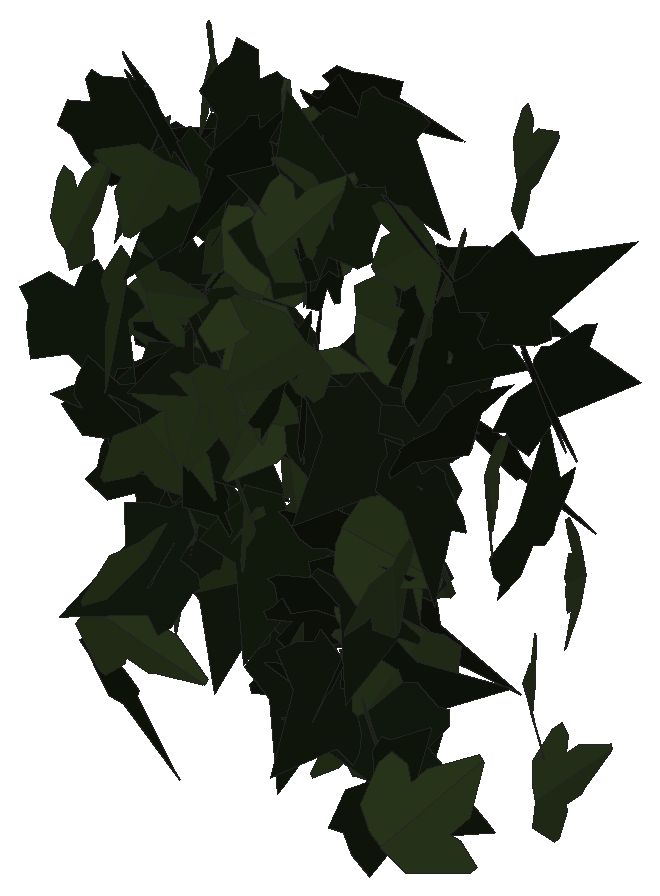
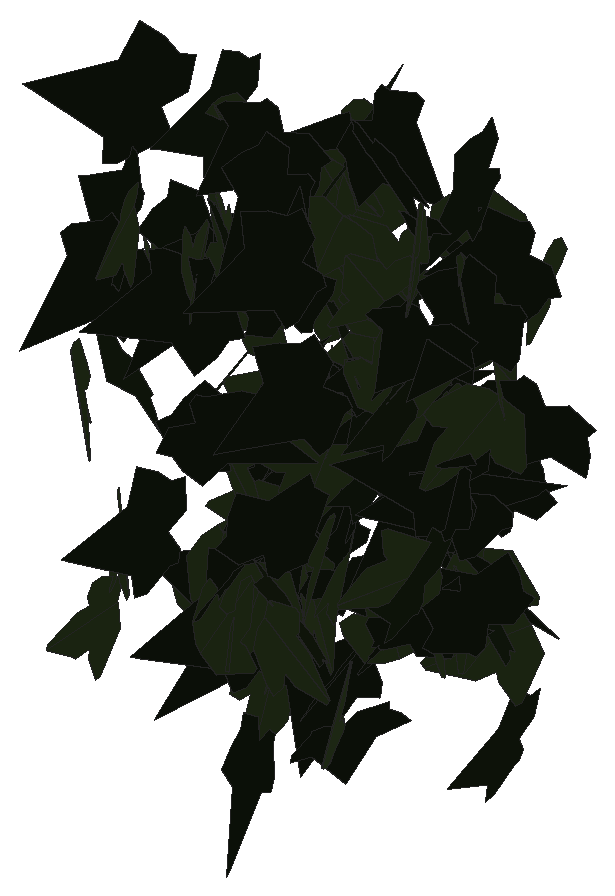
# SketchUp Ruby script. Lengths in inches.
U = 1.inch
M = Sketchup.active_model
def pt(a) = Geom::Point3d.new(a.map { |v| v * U })
def face(e, loops, mat)
  f = e.add_face(loops[0].map { |a| pt(a) })
  loops[1..].each { |l| e.add_face(l.map { |a| pt(a) }).erase! }
  f.material = f.back_material = mat if mat
  f
end
# faces: each face lists its corners as indices into pts; further lists are holes
def faces(e, pts, list, mat = nil) = list.each { |f| face(e, (f[0].is_a?(Array) ? f : [f]).map { |l| l.map { |i| pts[i] } }, mat) }
# xy, xz, yz: faces in a plane at the given z, y or x. An outline is a flat list of corners, or four numbers for a rectangle; further outlines are holes
def ring(l) = l.size == 4 ? [[l[0], l[1]], [l[2], l[1]], [l[2], l[3]], [l[0], l[3]]] : l.each_slice(2).to_a
def flat(e, list, mat, &to3) = list.each { |f| face(e, (f[0].is_a?(Array) ? f : [f]).map { |l| ring(l).map { |u, v| to3.(u, v) } }, mat) }
def xy(e, z, list, mat = nil) = flat(e, list, mat) { |x, y| [x, y, z] }
def xz(e, y, list, mat = nil) = flat(e, list, mat) { |x, z| [x, y, z] }
def yz(e, x, list, mat = nil) = flat(e, list, mat) { |y, z| [x, y, z] }
def lines(e, pts, list) = list.each { |a, b| e.add_line(pt(pts[a]), pt(pts[b])) }
# prism: a flat outline (further loops are holes) pulled along v
def prism(e, loops, v, mat = nil)
  f = face(e, loops, mat); d = Geom::Vector3d.new(v.map { |x| x * U })
  f.pushpull(f.normal.samedirection?(d) ? d.length : -d.length)
end
def box(e, o, s, mat = nil) = prism(e, [[o, [o[0] + s[0], o[1], o[2]], [o[0] + s[0], o[1] + s[1], o[2]], [o[0], o[1] + s[1], o[2]]]], [0, 0, s[2]], mat)
def at(x, y, z, deg = 0) = Geom::Transformation.translation(pt([x, y, z])) * Geom::Transformation.rotation(ORIGIN, Z_AXIS, deg.degrees)
def axes(o, x, y, z) = Geom::Transformation.new([*x, 0, *y, 0, *z, 0, *pt(o).to_a, 1])
def part(name) = M.definitions.add(name)
# library, detail: a bought-in or finely detailed component or shape, given as its bounding box
def library(name, o, s) = part(name).tap { |d| box(d.entities, o, s) }
def detail(e, o, s) = box(e.add_group.entities, o, s)
def put(e, d, t, mat = nil) = e.add_instance(d, t).tap { |i| i.material = mat if mat }
def group(e, t, mat = nil) = e.add_group.tap { |g| g.transformation = t; g.material = mat if mat }.entities
root = M.entities
M.materials.add("efeu1").color = [18, 25, 13]
M.materials.add("efeu2").color = [43, 57, 29]
c1 = part("ivyleaf_9")
p = [[1.54,2.16,1.25],[1.36,2.04,1.19],[-0.21,0.99,0.68],[-0.71,1.11,0.82],[-0.85,0.86,0.67],[-0.8,0.17,0.21],
  [-0.9,-0.01,0.1],[-0.67,-0.16,-0.02],[-0.08,-0.08,-0.05],[-0.03,-0.6,-0.4],[0.65,-0.88,-0.66],[0.83,-0.6,-0.49],
  [1.29,-0.42,-0.43],[1.8125,-0.07,-0.26],[1.21,0.44,0.15]]
faces(c1.entities,p,[[0,1,2,3,4,5,6,7,8,9,10,11,12,13,14]],"efeu1")
c2 = part("ivyleaf_10")
p = [[0,0.5,-0.03],[-0.0625,2.02,-0.43],[-0.19,2.01,-0.46],[-0.54,1.05,-0.29],[-0.52,0.625,-0.18],[-0.83,0.76,-0.28],
  [-1.16,0.64,-0.33],[-1.15,0.33,-0.24],[-0.77,-0.39,0.02],[-0.3,-0.51,0.16],[0.04,-0.48,0.23],[-0.02,2.01,-0.4375],
  [-0.06,2.01,-0.43],[0.04,-0.49,0.23],[0.67,-0.49,0.14],[1.38,0.36,-0.2],[1.375,0.51,-0.24],[0.81,0.65,-0.19],
  [0.62,0.59,-0.15],[0.6,1.09,-0.28],[0.5,1.23,-0.31]]
faces(c2.entities,p,[[0,1,2,3,4,5,6,7,8,9,10],[11,12,0,13,14,15,16,17,18,19,20]],"efeu2")
put(root,c1,axes([535.21,138.35,177.43],[0.48207,-0.59856,0.20369],[0.14027,-0.14851,-0.76839],[0.61651,0.50182,0.01555]))
put(root,c1,axes([535.3125,134.73,179.44],[-0.27899,-0.26925,-0.74167],[0.55413,0.49316,-0.38748],[0.56171,-0.62025,0.01388]))
put(root,c1,axes([535.34,135.23,182.82],[0.09988,-0.00032,-0.76274],[0.56999,0.51119,0.07443],[0.50683,-0.57483,0.06661]))
put(root,c1,axes([535.74,135.73,181.85],[0.51801,0.54955,0.22927],[0.14515,0.17819,-0.75505],[-0.5775,0.53773,0.01588]))
put(root,c2,axes([536.02,133.7,181.36],[0.0294,0.29057,-0.75135],[0.02416,0.75119,0.29146],[0.80521,-0.03315,0.01869]))
put(root,c1,axes([535.76,135.85,175.4],[-0.15333,-0.07864,0.76423],[0.70864,0.28655,0.17166],[-0.29677,0.72488,0.01505]))
put(root,c2,axes([535.86,137.66,177.16],[0.10862,0.11928,0.73924],[0.24864,0.69886,-0.1493],[-0.70632,0.26435,0.06113]))
put(root,c2,axes([536.05,135.42,181.02],[0.22066,-0.82498,0.09562],[-0.00156,0.09853,0.85365],[-0.83051,-0.21937,0.0238]))
put(root,c1,axes([535.81,134.89,172.53],[0.60317,-0.5162,0.04875],[0.03688,-0.03188,-0.7939],[0.51719,0.6043,-0.00024]))
put(root,c2,axes([536.13,135.38,179.3],[-0.52269,-0.40509,-0.52109],[0.39164,0.34468,-0.6608],[0.53127,-0.65264,-0.02555]))
put(root,c1,axes([536.88,135.8,177.53],[-0.42085,-0.08815,0.66579],[-0.62736,-0.22886,-0.42686],[0.23972,-0.75367,0.05175]))
put(root,c2,axes([536.5,135.43,182],[0.32264,-0.70335,-0.12966],[-0.06803,0.11142,-0.77367],[0.71196,0.32939,-0.01517]))
put(root,c1,axes([536.52,135.94,178.05],[0.62655,0.0255,-0.47755],[-0.4781,0.01515,-0.62647],[-0.01109,0.78765,0.02751]))
put(root,c1,axes([536.25,136.89,181.72],[-0.24445,-0.32961,-0.64417],[0.44367,0.46886,-0.40827],[0.57163,-0.50486,0.04141]))
put(root,c2,axes([536.68,136.55,183.5],[0.32496,-0.53129,-0.4965],[-0.05851,0.52295,-0.59789],[0.72482,0.28041,0.17433]))
put(root,c2,axes([536.27,134.6875,179.95],[0.26676,-0.48349,0.71737],[0.51173,-0.51709,-0.5388],[0.69751,0.56427,0.12093]))
put(root,c1,axes([536.1875,134.58,177.1],[-0.17328,0.05557,0.77942],[0.69673,-0.35045,0.17988],[0.35376,0.71743,0.0275]))
put(root,c1,axes([536.24,135.2,177.59],[0.4585,0.2321,0.66706],[0.55433,0.37457,-0.51134],[-0.43767,0.71756,0.05116]))
put(root,c1,axes([536.91,134.43,174.72],[-0.55418,0.52698,-0.25199],[-0.19513,0.16039,0.76454],[0.55058,0.58728,0.01732]))
put(root,c1,axes([537.2,136.13,174.625],[-0.6712,-0.43181,0.12924],[0.11128,0.0659,0.79809],[-0.43678,0.68034,0.00472]))
put(root,c1,axes([536.28,135.96,178.14],[0.41914,-0.00437,0.67662],[0.66741,0.13362,-0.41257],[-0.11133,0.78462,0.07403]))
put(root,c1,axes([536.67,134.73,183.85],[0.79047,-0.33972,-0.29967],[-0.27706,0.11427,-0.86037],[0.3584,0.83761,-0.00417]))
put(root,c1,axes([536.55,137.02,180.19],[0.60846,-0.46082,0.01006],[0.00814,-0.00592,-0.76327],[0.46086,0.60851,0.0002]))
put(root,c2,axes([537.34,134.36,182.62],[-0.64774,-0.28277,0.33722],[-0.29999,-0.15534,-0.70649],[0.322,-0.71356,0.02017]))
put(root,c2,axes([537.07,134.3125,175.25],[-0.32956,-0.7796,-0.26398],[0.09485,0.24649,-0.84636],[0.8176,-0.34284,-0.00822]))
put(root,c2,axes([536.7,134.04,174.02],[-0.50139,-0.05608,-0.73277],[0.72865,0.07765,-0.50451],[0.09576,-0.88448,0.00217]))
put(root,c1,axes([537.71,134.34,175.34],[-0.77582,0.09988,0.22816],[-0.22554,0.03492,-0.7822],[-0.10566,-0.80792,-0.0056]))
put(root,c2,axes([537.16,138.5,173.49],[-0.43688,0.49632,0.37938],[0.23325,-0.29987,0.6609],[0.57953,0.49484,0.01999]))
put(root,c2,axes([536.98,135.62,174.79],[0.14997,-0.35752,0.68886],[0.48487,-0.50468,-0.36749],[0.60602,0.49227,0.12355]))
put(root,c1,axes([537.0625,135.8,180.34],[0.16986,-0.77294,0.08753],[0.03334,-0.08228,-0.79125],[0.77717,0.17246,0.01481]))
put(root,c1,axes([537.21,135.625,177.28],[0.07653,-0.30387,-0.73011],[-0.08193,0.72653,-0.31096],[0.78657,0.10524,0.03864]))
put(root,c2,axes([537.34,134.36,177.6],[-0.58863,-0.52168,-0.42239],[0.3064,0.29103,-0.78643],[0.59723,-0.66348,-0.01284]))
put(root,c1,axes([537.81,134.95,182.39],[-0.75452,-0.03471,-0.10678],[0.1066,0.00634,-0.75531],[0.03525,-0.76201,-0.00142]))
put(root,c2,axes([538.15,138.92,175.61],[-0.28914,0.06197,0.75697],[-0.7595,-0.02019,-0.28846],[-0.00319,-0.81006,0.0651]))
put(root,c1,axes([537.3,135.76,176.37],[-0.09297,-0.36147,0.73067],[0.11384,-0.73396,-0.34861],[0.80721,0.06188,0.13332]))
put(root,c2,axes([537.58,136.59,181.84],[0.33475,0.52048,-0.44431],[0.14382,0.43007,0.61215],[0.66906,-0.35286,0.09072]))
put(root,c2,axes([537.26,134.39,180.24],[-0.31925,-0.02982,0.67465],[0.6753,-0.01782,0.31877],[0.00337,0.74616,0.03458]))
put(root,c2,axes([537.86,135.86,179.375],[-0.55956,-0.54167,-0.08654],[-0.06217,-0.0602,0.77879],[-0.54501,0.56301,0.00001]))
put(root,c1,axes([537.53,138.42,180.7],[0.55152,0.38294,0.36968],[0.2942,0.22432,-0.67127],[-0.44357,0.62491,0.01443]))
put(root,c1,axes([538.1,135.66,179],[-0.31822,-0.38007,0.62949],[-0.41315,-0.47499,-0.49564],[0.60828,-0.52144,-0.00733]))
put(root,c2,axes([538.12,134.62,178.51],[-0.63528,-0.46939,0.21211],[-0.16449,-0.13428,-0.78981],[0.48812,-0.65616,0.0099]))
put(root,c1,axes([537.77,137.39,173.17],[-0.16133,-0.73886,-0.15481],[0.04139,0.14941,-0.75622],[0.75377,-0.16634,0.00839]))
put(root,c1,axes([537.75,135.88,174.48],[-0.02758,-0.75428,0.24834],[0.01233,-0.24887,-0.75451],[0.79402,-0.02233,0.02035]))
put(root,c2,axes([537.93,135.8125,174.32],[-0.22665,-0.76206,0.03108],[0.00902,0.02974,0.79505],[-0.76264,0.22683,0.00017]))
put(root,c2,axes([538.03,137.08,176.33],[-0.22652,0.70891,-0.17425],[0.05019,-0.1669,-0.74422],[-0.72829,-0.23199,0.00291]))
put(root,c1,axes([538.6,135.14,181.42],[-0.40243,0.69705,-0.05013],[0.02332,-0.04442,-0.80488],[-0.69847,-0.4031,0.00201]))
put(root,c1,axes([538.32,139.2,173.39],[0.58308,-0.05687,-0.5647],[-0.55908,0.08188,-0.58551],[0.09775,0.80757,0.0196]))
put(root,c1,axes([538.41,135.64,184.12],[-0.71759,-0.02432,-0.39354],[0.39367,0.0014,-0.71793],[0.022,-0.81842,0.01047]))
put(root,c2,axes([538.49,137.04,176.72],[-0.37527,0.59932,0.29821],[-0.1666,0.2475,-0.70706],[-0.64835,-0.41048,0.00908]))
put(root,c1,axes([538.27,135.68,179.66],[-0.27054,-0.66992,-0.34937],[0.14247,0.3192,-0.72239],[0.74199,-0.30555,0.01132]))
put(root,c2,axes([538.39,135.17,181.12],[-0.0356,-0.80114,0.35276],[0.04212,0.35107,0.80156],[-0.87435,0.04953,0.02425]))
put(root,c1,axes([538.03,136.15,178.06],[0.68849,-0.34776,0.13065],[0.11743,-0.0573,-0.77133],[0.35245,0.69843,0.00178]))
put(root,c2,axes([538.11,135.6,175.89],[-0.24307,0.1456,0.75017],[0.64999,-0.37455,0.28331],[0.40183,0.69394,-0.00449]))
put(root,c1,axes([538.375,138.27,181.94],[0.72666,-0.22595,0.13053],[-0.11187,0.07917,0.75983],[-0.23575,-0.73403,0.04177]))
put(root,c1,axes([538.76,137.56,175.22],[-0.60002,0.53112,-0.11047],[-0.08388,0.0719,0.80131],[0.53596,0.60585,0.00175]))
put(root,c2,axes([538.58,135.34,179.75],[0.73585,0.25516,-0.0371],[-0.03489,-0.0126,-0.77883],[-0.25547,0.73668,-0.00047]))
put(root,c2,axes([538.84,134.62,178.9],[-0.81252,-0.26571,0.03952],[-0.03392,-0.02343,-0.85478],[0.26649,-0.81314,0.01171]))
put(root,c1,axes([538.7,136.15,175.51],[-0.46893,-0.66083,-0.07989],[0.0519,0.06113,-0.81028],[0.66361,-0.47175,0.00692]))
put(root,c1,axes([538.31,138.08,182.88],[0.69024,0.12291,0.31894],[0.30942,0.08065,-0.70073],[-0.14522,0.75608,0.02289]))
put(root,c2,axes([538.59,136.47,182.84],[0.66307,0.12344,0.36876],[0.36366,0.06138,-0.67444],[-0.13775,0.75623,-0.00545]))
put(root,c2,axes([538.75,136.71,178.08],[0.66801,0.55413,0.27162],[0.20168,0.18227,-0.86785],[-0.58323,0.6977,0.011]))
put(root,c1,axes([539.23,134.65,183.89],[-0.27295,0.41225,-0.65699],[0.2735,-0.60059,-0.49048],[-0.7258,-0.38135,0.06225]))
put(root,c2,axes([539.27,135.49,178.39],[0.32215,0.45864,-0.58428],[-0.34508,-0.47155,-0.56042],[-0.65776,0.47202,0.00785]))
put(root,c1,axes([539.4,137.59,176.36],[0.16866,0.16757,0.74554],[-0.67555,-0.32413,0.22568],[0.35713,-0.69225,0.0748]))
put(root,c1,axes([539.78,134.68,179.34],[-0.50634,0.20726,-0.59662],[-0.55145,0.22772,0.54712],[0.30792,0.74865,-0.00125]))
put(root,c1,axes([539.61,135.45,177.88],[-0.00423,-0.11342,0.82894],[0.03828,0.82806,0.11349],[-0.83579,0.0385,0.001]))
put(root,c1,axes([539.27,135.79,172.98],[0.01145,-0.7154,0.3866],[0.00024,-0.38663,-0.71547],[0.81317,0.01019,-0.00523]))
put(root,c1,axes([539.59,135.48,173.33],[0.53867,0.54518,-0.24257],[-0.18677,-0.15633,-0.7661],[-0.56673,0.56971,0.02191]))
put(root,c2,axes([540.14,134.43,180.23],[-0.56354,-0.19468,0.67021],[-0.6415,-0.1948,-0.59598],[0.27489,-0.85371,-0.01684]))
put(root,c1,axes([539.21,135.5,178.73],[-0.31764,-0.24491,-0.71185],[0.55927,0.44041,-0.40108],[0.50391,-0.64316,-0.00357]))
put(root,c1,axes([538.97,135.45,177.92],[0.4578,0.03447,0.66244],[0.66272,0.01109,-0.45857],[-0.02873,0.80516,-0.02205]))
put(root,c2,axes([539.75,135.79,174.7],[0.26251,-0.78838,0.02196],[0.00957,-0.01996,-0.83093],[0.78863,0.26267,0.00277]))
put(root,c1,axes([540.16,138.53,179.09],[-0.04839,-0.12472,-0.7707],[-0.2387,-0.73284,0.13358],[-0.74334,0.24345,0.00728]))
put(root,c2,axes([539.8,137.2,175.29],[-0.21099,-0.64049,-0.40511],[0.17151,0.36925,-0.67312],[0.73819,-0.26886,0.04061]))
put(root,c2,axes([540.34,134.7,182.86],[0.28653,-0.07436,-0.73317],[-0.6733,0.29334,-0.29289],[0.29955,0.73047,0.04298]))
put(root,c2,axes([539.67,134.51,181.59],[0.56628,0.63153,-0.45624],[0.30901,0.3357,0.84822],[0.71519,-0.64508,-0.00524]))
put(root,c2,axes([540.13,134.73,182.32],[0.52339,-0.43675,-0.50405],[-0.27374,0.44359,-0.66861],[0.60817,0.57552,0.13283]))
put(root,c2,axes([540.33,137.92,174.375],[-0.654,0.22592,-0.36703],[-0.35496,0.09597,0.69156],[0.24444,0.74379,0.02225]))
put(root,c1,axes([539.87,136.5,183.37],[0.74794,0.1255,-0.16887],[-0.16967,-0.00897,-0.75817],[-0.12441,0.76672,0.01877]))
put(root,c1,axes([540.08,134.98,182.51],[0.41842,-0.76132,-0.18772],[0.10427,-0.15686,0.86858],[-0.77716,-0.43094,0.01546]))
put(root,c2,axes([540.72,136.88,177.48],[0.27348,-0.23363,-0.69617],[-0.51346,0.47024,-0.35952],[0.52496,0.58165,0.01103]))
put(root,c1,axes([540.84,134.45,182.34],[-0.93262,-0.15857,0.03687],[0.03891,-0.00889,0.94588],[-0.15808,0.93331,0.01528]))
put(root,c1,axes([540.58,134.79,181.53],[-0.05865,-0.44691,0.68422],[0.12865,0.67238,0.4502],[-0.80705,0.13966,0.02204]))
put(root,c1,axes([539.98,134.81,174.82],[0.33542,0.66325,-0.38538],[0.11119,0.37413,0.74067],[0.75898,-0.34792,0.06181]))
put(root,c1,axes([540.11,135.07,176.66],[0.80048,0.12027,0.1186],[0.11768,0.01495,-0.80946],[-0.12117,0.80908,-0.00268]))
put(root,c1,axes([541.08,137.41,177.9],[-0.1455,-0.0176,0.81186],[-0.76251,-0.28071,-0.14274],[0.27929,-0.77556,0.03324]))
put(root,c2,axes([540.69,135.68,172.65],[-0.2947,-0.69889,-0.32573],[0.1277,0.29965,-0.75848],[0.76042,-0.32118,0.00114]))
put(root,c2,axes([540.49,133.72,182.7],[0.18281,0.24503,-0.78762],[0.3369,0.7142,0.30038],[0.75292,-0.37907,0.05683]))
put(root,c1,axes([540.97,134.34,173.99],[-0.04136,0.52449,0.64819],[-0.04231,0.64683,-0.52609],[-0.83274,-0.05891,-0.00546]))
put(root,c1,axes([540.42,136.69,175.18],[0.26175,-0.78826,-0.38897],[-0.12755,0.36749,-0.83057],[0.8697,0.29113,-0.00475]))
put(root,c1,axes([540.72,134.91,173.6875],[-0.1619,-0.59527,0.53616],[-0.1437,-0.51655,-0.61689],[0.78814,-0.21646,-0.00234]))
put(root,c1,axes([540.35,136.01,183.9],[-0.15796,-0.19176,-0.79434],[0.539,0.58364,-0.24807],[0.61419,-0.5615,0.01342]))
put(root,c1,axes([540.89,135.68,178.27],[-0.26781,-0.6092,0.50502],[-0.17899,-0.47271,-0.66513],[0.7708,-0.32143,0.02101]))
put(root,c1,axes([540.27,136.8,174.32],[0.82716,-0.12645,0.37067],[0.36385,-0.07239,-0.83663],[0.14491,0.90352,-0.01516]))
put(root,c2,axes([540.89,135.44,173.17],[-0.50994,0.62916,-0.16703],[0.1045,-0.13031,-0.80986],[-0.64251,-0.52054,0.00085]))
put(root,c1,axes([540.82,134.26,176.12],[0.78009,0.50436,0.10851],[0.09018,0.06037,-0.92893],[-0.50796,0.78528,0.00172]))
put(root,c1,axes([541.47,136.8,177.49],[-0.25114,-0.70114,-0.25858],[-0.04679,-0.2575,0.74366],[-0.74583,0.25224,0.04041]))
put(root,c2,axes([540.5,136.15,180.07],[-0.01444,0.00361,0.82843],[0.8136,0.15616,0.0135],[-0.15608,0.81371,-0.00627]))
put(root,c2,axes([540.9375,135.51,175.86],[0.32333,0.65749,0.38819],[0.14363,0.36166,-0.73219],[-0.74991,0.35275,0.02714]))
put(root,c1,axes([540.78,138.8125,176.79],[0.71511,-0.29359,0.30538],[0.28765,-0.10333,-0.77292],[0.31098,0.77069,0.0127]))
put(root,c2,axes([541.84,135.55,174.62],[-0.53315,-0.60408,0.47024],[-0.31521,-0.34899,-0.80569],[0.69762,-0.61934,-0.00466]))
put(root,c1,axes([541.85,135.47,180.68],[-0.05887,0.32372,0.73238],[-0.19193,0.70724,-0.32804],[-0.77739,-0.19913,0.02553]))
put(root,c1,axes([542.26,135.25,172.98],[-0.39136,-0.27666,-0.767],[-0.6253,-0.44417,0.47927],[-0.52328,0.73768,0.00092]))
put(root,c1,axes([541.4,135.23,175.875],[-0.10118,-0.76423,0.26964],[-0.045,-0.26602,-0.77085],[0.80916,-0.11036,-0.00915]))
put(root,c2,axes([541.47,137.17,180.89],[0.05486,-0.16322,-0.77629],[0.19316,-0.75197,0.17176],[-0.76938,-0.20042,-0.01224]))
put(root,c1,axes([541.22,137.14,180.75],[0.08642,0.11215,-0.81339],[0.4462,0.68017,0.14119],[0.68927,-0.45437,0.01059]))
put(root,c2,axes([541.95,138.29,182.57],[0.06719,-0.15203,-0.82381],[-0.07418,0.82213,-0.15777],[0.83443,0.08533,0.05231]))
put(root,c1,axes([541.28,135.47,173.75],[0.34471,-0.1407,0.72585],[0.72639,-0.08487,-0.36142],[0.13785,0.79905,0.08942]))
put(root,c2,axes([541.8125,134.29,177.1875],[0.08195,0.53616,0.69382],[0.12362,0.68282,-0.54226],[-0.86808,0.14785,-0.01172]))
put(root,c1,axes([542.12,135.79,180.52],[0.00202,-0.03525,-0.90722],[-0.3766,0.82546,-0.03291],[0.82611,0.37639,-0.01279]))
put(root,c2,axes([542.51,134.8,182.84],[0.53992,-0.15425,-0.6199],[-0.51647,0.37225,-0.54246],[0.37593,0.73295,0.14504]))
put(root,c2,axes([542.28,134.38,176.63],[-0.01484,-0.78479,-0.29344],[-0.01177,0.29365,-0.78476],[0.83777,-0.00977,-0.01622]))
put(root,c1,axes([542.05,134.38,172.62],[0.14856,-0.10795,-0.88524],[-0.20482,0.86931,-0.14039],[0.86795,0.22362,0.11839]))
put(root,c2,axes([542.23,135.1,180.33],[0.41079,-0.71874,-0.00644],[0.00413,-0.00506,0.82785],[-0.71876,-0.41081,0.00108]))
put(root,c1,axes([542.08,135.48,177.94],[0.18388,-0.75119,0.21431],[0.049,-0.20864,-0.77337],[0.77962,0.19029,-0.00194]))
put(root,c1,axes([542.31,134.82,183.2],[0.69332,-0.47552,0.18356],[0.1541,-0.09985,-0.84071],[0.48587,0.71022,0.0047]))
put(root,c2,axes([542.72,134.17,172.1],[0.65718,0.14401,-0.65962],[0.64613,0.13287,0.67275],[0.19585,-0.92159,-0.00608]))
put(root,c1,axes([543.55,134.05,180.04],[0.13876,0.83297,0.17081],[0.02859,0.1684,-0.84445],[-0.84982,0.14167,-0.00052]))
put(root,c2,axes([544.34,135.67,174.25],[-0.14485,0.11536,0.83732],[-0.70705,0.44895,-0.18417],[-0.46314,-0.72148,0.01928]))
put(root,c1,axes([544.02,136.17,180.18],[-0.08065,0.15868,-0.8708],[-0.30943,0.81418,0.17702],[0.82929,0.31922,-0.01864]))
put(root,c1,axes([544.54,135.36,177.69],[-0.65814,0.3832,-0.52809],[-0.45718,0.26432,0.76157],[0.46551,0.80135,0.00133]))
put(root,c2,axes([544.01,134.93,178.79],[0.02802,-0.16305,-0.82191],[0.38237,-0.72927,0.15771],[-0.7456,-0.38012,0.04999]))
put(root,c2,axes([544.36,135.97,172.62],[0.01808,-0.02662,-0.82961],[0.17522,0.81123,-0.02221],[0.81133,-0.1746,0.02328]))
put(root,c1,axes([543.99,135.89,180.71],[0.39918,-0.04846,-0.86177],[0.8527,-0.12509,0.40201],[-0.13384,-0.94146,-0.00905]))
put(root,c1,axes([544.41,134.51,182.43],[0.16524,0.12876,0.87724],[0.77243,0.41719,-0.20673],[-0.43529,0.78918,-0.03384]))
put(root,c2,axes([545.25,135.65,177.14],[0.29063,-0.41594,-0.70162],[-0.36052,0.60261,-0.50658],[0.73165,0.46216,0.02908]))
